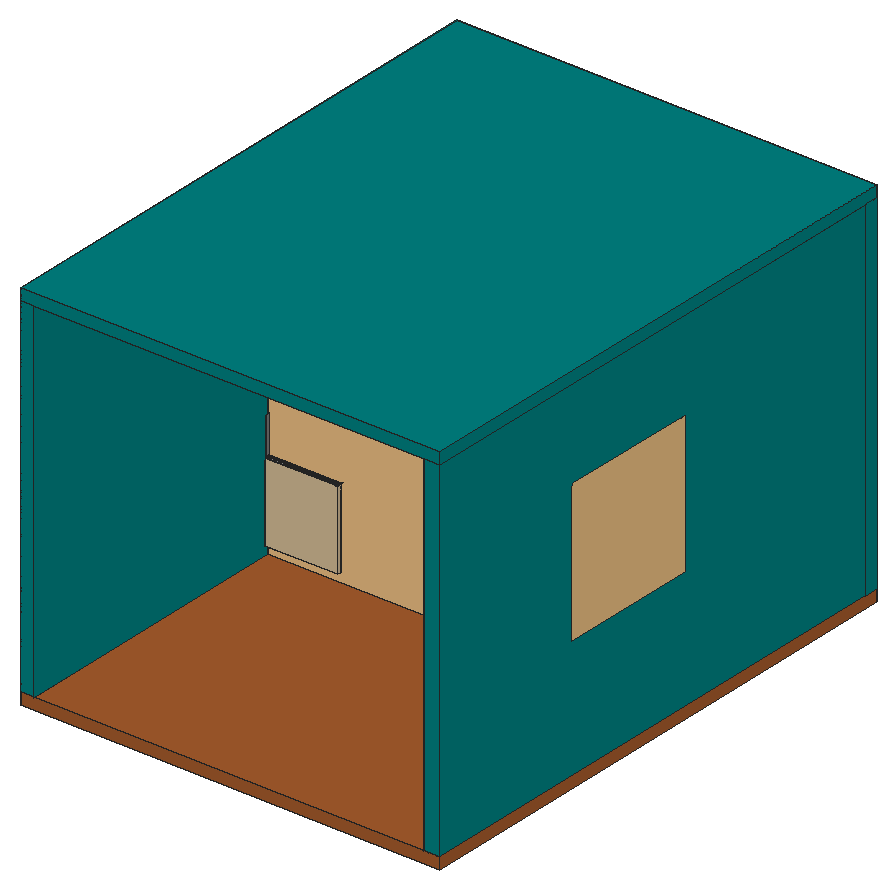
# SketchUp Ruby script. Lengths in inches.
U = 1.inch
M = Sketchup.active_model
def pt(a) = Geom::Point3d.new(a.map { |v| v * U })
def face(e, loops, mat)
  f = e.add_face(loops[0].map { |a| pt(a) })
  loops[1..].each { |l| e.add_face(l.map { |a| pt(a) }).erase! }
  f.material = f.back_material = mat if mat
  f
end
# faces: each face lists its corners as indices into pts; further lists are holes
def faces(e, pts, list, mat = nil) = list.each { |f| face(e, (f[0].is_a?(Array) ? f : [f]).map { |l| l.map { |i| pts[i] } }, mat) }
# xy, xz, yz: faces in a plane at the given z, y or x. An outline is a flat list of corners, or four numbers for a rectangle; further outlines are holes
def ring(l) = l.size == 4 ? [[l[0], l[1]], [l[2], l[1]], [l[2], l[3]], [l[0], l[3]]] : l.each_slice(2).to_a
def flat(e, list, mat, &to3) = list.each { |f| face(e, (f[0].is_a?(Array) ? f : [f]).map { |l| ring(l).map { |u, v| to3.(u, v) } }, mat) }
def xy(e, z, list, mat = nil) = flat(e, list, mat) { |x, y| [x, y, z] }
def xz(e, y, list, mat = nil) = flat(e, list, mat) { |x, z| [x, y, z] }
def yz(e, x, list, mat = nil) = flat(e, list, mat) { |y, z| [x, y, z] }
def lines(e, pts, list) = list.each { |a, b| e.add_line(pt(pts[a]), pt(pts[b])) }
# prism: a flat outline (further loops are holes) pulled along v
def prism(e, loops, v, mat = nil)
  f = face(e, loops, mat); d = Geom::Vector3d.new(v.map { |x| x * U })
  f.pushpull(f.normal.samedirection?(d) ? d.length : -d.length)
end
def box(e, o, s, mat = nil) = prism(e, [[o, [o[0] + s[0], o[1], o[2]], [o[0] + s[0], o[1] + s[1], o[2]], [o[0], o[1] + s[1], o[2]]]], [0, 0, s[2]], mat)
def at(x, y, z, deg = 0) = Geom::Transformation.translation(pt([x, y, z])) * Geom::Transformation.rotation(ORIGIN, Z_AXIS, deg.degrees)
def axes(o, x, y, z) = Geom::Transformation.new([*x, 0, *y, 0, *z, 0, *pt(o).to_a, 1])
def part(name) = M.definitions.add(name)
# library, detail: a bought-in or finely detailed component or shape, given as its bounding box
def library(name, o, s) = part(name).tap { |d| box(d.entities, o, s) }
def detail(e, o, s) = box(e.add_group.entities, o, s)
def put(e, d, t, mat = nil) = e.add_instance(d, t).tap { |i| i.material = mat if mat }
def group(e, t, mat = nil) = e.add_group.tap { |g| g.transformation = t; g.material = mat if mat }.entities
root = M.entities
M.materials.add("CLC2-PC-Blanc INTER").color = [249, 249, 249]
M.materials.add("Material \#1").color = [0, 0, 0]
M.materials.add("Standardmaterial30").color = [86, 86, 86]
M.materials.add("[0031_PapayaWhip]").color = [199, 195, 183]
M.materials.add("[0031_PapayaWhip]1").color = [211, 117, 3]
M.materials.add("[0079_Teal]").color = [0, 128, 128]
M.materials.add("[0088_Aquamarine]").color = [127, 255, 212]
M.materials.add("[0091_MintCream]").color = [201, 113, 3]
M.materials.add("[0099_LightSteelBlue]").color = [176, 196, 222]
M.materials.add("[Blacktop Old 01]").color = [132, 136, 139]
M.materials.add("[Blinds Wood White]").color = [138, 137, 139]
M.materials.add("[Encaustic Tile Circular 01]").color = [123, 123, 122]
M.materials.add("[Formica Beige]").color = [211, 187, 149]
M.materials.add("[Ornate Tile 01]").color = [202, 202, 202]
M.materials.add("[Resin Turquoise]").color = [117, 218, 223]
M.materials.add("[Stone Marble]").color = [143, 138, 136]
M.materials.add("[Stone Vein Gray]").color = [166, 165, 165]
M.materials.add("[Terrazzo Light Blue]").color = [196, 214, 227]
M.materials.add("[Tile Hexagon White]").color = [213, 206, 204]
M.materials.add("[Translucent Glass Gray]").color = [128, 128, 128]
M.materials["[Translucent Glass Gray]"].alpha = 0.5
M.materials.add("[Wood Board Cork]").color = [215, 201, 115]
M.materials.add("[Wood Cherry Original]").color = [152, 86, 42]
M.materials.add("[Wood Square Tile 01]").color = [164, 91, 44]
M.materials.add("utensils_wood_2").color = [89, 58, 24]
c1 = library("Group\#12",[-32.31,-359.75,0.0625],[113.14,110.83,100])
c2 = library("Group\#19",[-370.5625,-274.21,5.8125],[90.77,166.34,120.375])
c3 = library("Group\#17",[-278.11,-348.23,5.8],[187.87,187.87,121.65])
c4 = library("Group\#13",[-77.16,-243.45,0.06],[77.78,77.39,334.5])
c5 = library("Group\#11",[5.16,-238.13,0.06],[77.38,77.77,330.87])
c6 = library("Group\#21",[162.6875,-473.8,0.53],[157.34,166.37,329.78])
c7 = library("Group\#14",[-424.81,-54.29,0.29],[386.66,43.55,222.03])
c8 = library("Group\#20",[70.49,-356.56,0.0625],[143.03,166.7,314.72])
c9 = library("Group\#22",[-91.3125,-441.93,-0.01],[120,70.11,138.07])
c10 = library("Group\#16",[-375.96,-353.73,0.05],[297.45,297.44,31.27])
c11 = library("Group\#18",[-284.5,-166.25,5.875],[106.63,106.63,250.48])
c12 = part("Kitchen countertop accessories")
p = [[424.81,473.8,0.01],[425.81,473.8,0.01],[425.81,474.8,0.01]]
lines(c12.entities,p,[[0,1],[2,0]])
put(c12.entities,c1,at(424.81,473.8,0.01))
put(c12.entities,c2,at(424.81,473.8,0.01))
put(c12.entities,c3,at(424.81,473.8,0.01))
put(c12.entities,c4,at(424.81,473.8,0.01))
put(c12.entities,c5,at(424.81,473.8,0.01))
put(c12.entities,c6,at(424.81,473.8,0.01))
put(c12.entities,c7,at(424.81,473.8,0.01),"utensils_wood_2")
put(c12.entities,c8,at(424.81,473.8,0.01))
put(c12.entities,c9,at(424.81,473.8,0.01))
put(c12.entities,c10,at(424.81,473.8,0.01))
put(c12.entities,c11,at(424.81,473.8,0.01))
c13 = library("pellawindow\#4",[0,-3.05,0],[47.5,4.65,53.5])
c14 = library("007",[-28.95,-65.99,21.26],[5.48,1.13,0.69])
c15 = library("5-HOTTE ASPIRANTE CLC2",[-15.16,-17.72,-0.29],[30.34,17.72,30.09])
c16 = library("Hob1",[-15.52,-17.72,0],[31.04,35.44,3.4])
c17 = library("6-FOUR H60 CLC2",[0,-1.15,0],[23.5,21.54,23.5])
c18 = library("2-TABLE DE CUISSON CLC2",[-11.42,-10.04,0],[22.84,20.08,1.26])
c19 = part("CLC2-Ele02")
prism(c19.entities,[[[0.84,-0.32,0.16],[0.84,-0.33,0.02],[0.84,-0.34,-0.125],[0.84,-0.36,-0.27],[0.84,-0.39,-0.41],[0.84,-0.43,-0.55],[0.84,-0.47,-0.68],[0.84,-0.51,-0.82],[0.84,-0.2,-0.84],[0.84,-0.07,0.84],[0.84,-0.375,0.87],[0.84,-0.35,0.73],[0.84,-0.33,0.59],[0.84,-0.32,0.44],[0.84,-0.32,0.3]]],[-0.83,0,0],"CLC2-PC-Blanc INTER")
prism(c19.entities,[[[-0.01,-0.32,0.16],[-0.01,-0.33,0.02],[-0.01,-0.34,-0.125],[-0.01,-0.36,-0.27],[-0.01,-0.39,-0.41],[-0.01,-0.43,-0.55],[-0.01,-0.47,-0.68],[-0.01,-0.51,-0.82],[-0.01,-0.2,-0.84],[-0.01,-0.07,0.84],[-0.01,-0.375,0.87],[-0.01,-0.35,0.73],[-0.01,-0.33,0.59],[-0.01,-0.32,0.44],[-0.01,-0.32,0.3]]],[-0.83,0,0],"CLC2-PC-Blanc INTER")
xy(c19.entities,-1.57,[[-1.44,-0.19,1.44,0]],"CLC2-PC-Blanc INTER")
xy(c19.entities,-1.5,[[-1.375,-0.12,1.375,0]],"CLC2-PC-Blanc INTER")
xy(c19.entities,-0.87,[[-0.85,-0.29,0.85,-0.12]],"CLC2-PC-Blanc INTER")
xy(c19.entities,0.87,[[-0.85,-0.29,0.85,-0.12]],"CLC2-PC-Blanc INTER")
xy(c19.entities,1.5,[[-1.375,-0.12,1.375,0]],"CLC2-PC-Blanc INTER")
xy(c19.entities,1.57,[[-1.44,-0.19,1.44,0]],"CLC2-PC-Blanc INTER")
xz(c19.entities,-0.12,[[[-1.375,-1.5,-1.41,-1.3,-1.4375,-1.04,-1.46,-0.78,-1.48,-0.52,-1.5,0,-1.48,0.52,-1.46,0.78,-1.4375,1.04,-1.41,1.3,-1.375,1.5,1.375,1.5,1.41,1.3,1.4375,1.04,1.46,0.78,1.48,0.52,1.5,0,1.48,-0.52,1.46,-0.78,1.4375,-1.04,1.41,-1.3,1.375,-1.5],[-0.85,-0.87,0.85,0.87]]],"CLC2-PC-Blanc INTER")
xz(c19.entities,0,[[-1.44,-1.57,-1.48,-1.3125,-1.51,-1.05,-1.54,-0.79,-1.56,-0.53,-1.57,-0.26,-1.57,0.26,-1.56,0.53,-1.54,0.79,-1.51,1.05,-1.48,1.3125,-1.44,1.57,0,1.57,0,1.5,-1.375,1.5,-1.41,1.3,-1.4375,1.04,-1.46,0.78,-1.48,0.52,-1.5,0,-1.48,-0.52,-1.46,-0.78,-1.4375,-1.04,-1.41,-1.3,-1.375,-1.5,0,-1.5,0,-1.57],[0,-1.57,0,-1.5,1.375,-1.5,1.41,-1.3,1.4375,-1.04,1.46,-0.78,1.48,-0.52,1.5,0,1.48,0.52,1.46,0.78,1.4375,1.04,1.41,1.3,1.375,1.5,0,1.5,0,1.57,1.44,1.57,1.48,1.3125,1.51,1.05,1.54,0.79,1.56,0.53,1.57,0.26,1.57,-0.26,1.56,-0.53,1.54,-0.79,1.51,-1.05,1.48,-1.3125,1.44,-1.57]],"CLC2-PC-Blanc INTER")
yz(c19.entities,-1.57,[[-0.0625,-0.26,-0.06,0,0,0,0,-0.26],[-0.06,0,-0.0625,0.26,0,0.26,0,0]],"CLC2-PC-Blanc INTER")
yz(c19.entities,-0.85,[[-0.29,-0.87,-0.12,-0.87,-0.12,0.87,-0.29,0.87,-0.29,0.79,-0.3125,0.53,-0.32,0.26,-0.33,0,-0.32,-0.26,-0.3125,-0.53,-0.29,-0.79]],"CLC2-PC-Blanc INTER")
yz(c19.entities,0.85,[[-0.29,-0.87,-0.29,-0.79,-0.3125,-0.53,-0.32,-0.26,-0.33,0,-0.32,0.26,-0.3125,0.53,-0.29,0.79,-0.29,0.87,-0.12,0.87,-0.12,-0.87]],"CLC2-PC-Blanc INTER")
yz(c19.entities,1.57,[[-0.0625,-0.26,0,-0.26,0,0,-0.06,0],[-0.06,0,0,0,0,0.26,-0.0625,0.26]],"CLC2-PC-Blanc INTER")
p = [[-1.32,-0.3125,0.53],[-1.34,-0.29,0.79],[-1.37,-0.27,1.05],[-1.4,-0.23,1.3125],[-1.44,-0.19,1.57],[-1.48,-0.15,1.3125],
  [-1.51,-0.12,1.05],[-1.54,-0.09,0.79],[-1.56,-0.07,0.53],[-1.57,-0.0625,0.26],[-1.57,-0.06,0],[-1.57,-0.0625,-0.26],
  [-1.56,-0.07,-0.53],[-1.54,-0.09,-0.79],[-1.51,-0.12,-1.05],[-1.48,-0.15,-1.3125],[-1.44,-0.19,-1.57],[-1.4,-0.23,-1.3125],
  [-1.37,-0.27,-1.05],[-1.34,-0.29,-0.79],[-1.32,-0.3125,-0.53],[-1.31,-0.32,-0.26],[-1.3,-0.33,0],[-1.31,-0.32,0.26],
  [1.34,-0.29,0.79],[1.32,-0.3125,0.53],[1.31,-0.32,0.26],[1.3,-0.33,0],[1.31,-0.32,-0.26],[1.32,-0.3125,-0.53],
  [1.34,-0.29,-0.79],[1.37,-0.27,-1.05],[1.4,-0.23,-1.3125],[1.44,-0.19,-1.57],[1.48,-0.15,-1.3125],[1.51,-0.12,-1.05],
  [1.54,-0.09,-0.79],[1.56,-0.07,-0.53],[1.57,-0.0625,-0.26],[1.57,-0.06,0],[1.57,-0.0625,0.26],[1.56,-0.07,0.53],
  [1.54,-0.09,0.79],[1.51,-0.12,1.05],[1.48,-0.15,1.3125],[1.44,-0.19,1.57],[1.4,-0.23,1.3125],[1.37,-0.27,1.05],
  [-1.44,0,-1.57],[-1.48,0,-1.3125],[1.44,0,-1.57],[1.48,0,-1.3125],[-1.375,0,-1.5],[-1.41,0,-1.3],
  [-1.41,-0.12,-1.3],[-1.375,-0.12,-1.5],[1.41,0,-1.3],[1.375,0,-1.5],[1.375,-0.12,-1.5],[1.41,-0.12,-1.3],
  [-1.51,0,-1.05],[1.51,0,-1.05],[-1.4375,0,-1.04],[-1.4375,-0.12,-1.04],[1.4375,0,-1.04],[1.4375,-0.12,-1.04],
  [0.85,-0.29,-0.87],[-0.85,-0.29,-0.87],[-0.85,-0.29,-0.79],[-1.33,-0.29,-0.79],[1.33,-0.29,-0.79],[0.85,-0.29,-0.79],
  [-1.54,0,-0.79],[1.54,0,-0.79],[-1.46,0,-0.78],[-1.46,-0.12,-0.78],[1.46,0,-0.78],[1.46,-0.12,-0.78],
  [-0.85,-0.3125,-0.53],[0.85,-0.3125,-0.53],[-1.56,0,-0.53],[-1.48,0,-0.52],[-1.48,-0.12,-0.52],[1.48,0,-0.52],
  [1.48,-0.12,-0.52],[1.56,0,-0.53],[-0.85,-0.32,-0.26],[0.85,-0.32,-0.26],[-1.57,0,-0.26],[-1.49,0,-0.26],
  [-1.49,-0.12,-0.26],[1.49,0,-0.26],[1.49,-0.12,-0.26],[1.57,0,-0.26],[-0.85,-0.33,0],[0.85,-0.33,0],
  [-1.5,0,0],[-1.5,-0.12,0],[1.5,0,0],[1.5,-0.12,0],[-0.85,-0.32,0.26],[0.85,-0.32,0.26],
  [-1.49,0,0.26],[-1.49,-0.12,0.26],[1.49,0,0.26],[1.49,-0.12,0.26],[-0.85,-0.3125,0.53],[0.85,-0.3125,0.53],
  [-1.57,0,0.26],[-1.56,0,0.53],[-1.48,0,0.52],[-1.48,-0.12,0.52],[1.48,0,0.52],[1.48,-0.12,0.52],
  [1.57,0,0.26],[1.56,0,0.53],[-0.85,-0.29,0.79],[-1.33,-0.29,0.79],[1.33,-0.29,0.79],[0.85,-0.29,0.79],
  [-1.54,0,0.79],[-1.46,0,0.78],[-1.46,-0.12,0.78],[1.46,0,0.78],[1.46,-0.12,0.78],[1.54,0,0.79],
  [-0.85,-0.29,0.87],[0.85,-0.29,0.87],[-1.4375,0,1.04],[-1.4375,-0.12,1.04],[-1.51,0,1.05],[1.4375,0,1.04],
  [1.4375,-0.12,1.04],[1.51,0,1.05],[-1.41,0,1.3],[-1.41,-0.12,1.3],[1.41,0,1.3],[1.41,-0.12,1.3],
  [-1.48,0,1.3125],[1.48,0,1.3125],[-1.44,0,1.57],[1.44,0,1.57],[-1.375,0,1.5],[-1.375,-0.12,1.5],
  [1.375,0,1.5],[1.375,-0.12,1.5]]
faces(c19.entities,p,[[0,1,2,3,4,5,6,7,8,9,10,11,12,13,14,15,16,17,18,19,20,21,22,23],[24,25,26,27,28,29,30,31,32,33,34,35,36,37,38,39,40,41,42,43,44,45,46,47],[48,16,15,49],[32,17,16,33],[33,50,51,34],[52,53,54,55],[56,57,58,59],[31,18,17,32],
  [49,15,14,60],[34,51,61,35],[53,62,63,54],[64,56,59,65],[66,67,68,69,19,18,31,30,70,71],[60,14,13,72],[35,61,73,36],[62,74,75,63],
  [76,64,65,77],[69,68,78,20,19],[71,70,30,29,79],[72,13,12,80],[74,81,82,75],[83,76,77,84],[36,73,85,37],[20,78,86,21],
  [79,29,28,87],[80,12,11,88],[81,89,90,82],[91,83,84,92],[37,85,93,38],[21,86,94,22],[87,28,27,95],[89,96,97,90],
  [98,91,92,99],[22,94,100,23],[95,27,26,101],[96,102,103,97],[104,98,99,105],[23,100,106,0],[101,26,25,107],[108,9,8,109],
  [102,110,111,103],[112,104,105,113],[40,114,115,41],[0,106,116,117,1],[107,25,24,118,119],[109,8,7,120],[110,121,122,111],[123,112,113,124],
  [41,115,125,42],[116,126,127,119,118,24,47,2,1,117],[121,128,129,122],[120,7,6,130],[131,123,124,132],[42,125,133,43],[128,134,135,129],[136,131,132,137],
  [46,3,2,47],[130,6,5,138],[43,133,139,44],[138,5,4,140],[4,3,46,45],[44,139,141,45],[134,142,143,135],[144,136,137,145]],"CLC2-PC-Blanc INTER")
c20 = part("2-PRISEELC CLC2")
put(c20.entities,c19,axes([0,0,0],[1,0,0],[0,0,-1],[0,1,0]))
c21 = library("15-PRODUITS CUISINE CLC2",[-1.94,-2.15,0],[3.93,3.94,5.51])
c22 = library("12-PRODUITS CUISINE CLC2",[-1.08,-1.08,0],[2.16,2.16,5.375])
c23 = library("15-PRODUITS CUISINE CLC2\#1",[-1.94,-2.15,0],[3.93,3.94,5.51])
c24 = library("Kitchen sink with faucet",[-0.15,-0.12,-6.4],[37.85,20.23,20.6])
c25 = library("AS-120-mm",[0,0,0],[48,4.72,48])
c26 = library("9-POIGNEE CLC2",[-3.01,-0.26,0],[6.02,0.52,1.49])
c27 = library("2-POIGNEE CLC2",[-2.66,-0.49,0],[5.32,0.98,1.3])
c28 = library("Group\#4",[0,32.625,0],[131,82,57])
c29 = part("Union")
xy(c29.entities,0,[[0,51.67,0.1,82.93]],"[Tile Hexagon White]")
xy(c29.entities,0.04,[[0.1875,0,0,51.67,0.1,51.67,0.29,0]],"[Tile Hexagon White]")
xy(c29.entities,12.44,[[0.1875,0,0.29,0,0.1,51.67,0,51.67]],"[Tile Hexagon White]")
xy(c29.entities,29.375,[[0,51.67,0.1,82.93]],"[Tile Hexagon White]")
xz(c29.entities,0,[[0.1875,0.04,0.29,12.44]],"[Tile Hexagon White]")
xz(c29.entities,51.67,[[0,0,0.1,0.04],[0,12.44,0.1,29.375]],"[Tile Hexagon White]")
xz(c29.entities,82.93,[[0,0,0.1,29.375]],"[Tile Hexagon White]")
yz(c29.entities,0,[[51.67,0,82.93,29.375]],"[Tile Hexagon White]")
yz(c29.entities,0.1,[[51.67,0,82.93,29.375]],"[Encaustic Tile Circular 01]")
p = [[0,51.67,0.04],[0.1875,0,0.04],[0.1875,0,12.44],[0,51.67,12.44],[0.29,0,0.04],[0.1,51.67,0.04],
  [0.1,51.67,12.44],[0.29,0,12.44]]
faces(c29.entities,p,[[0,1,2,3]],"[Tile Hexagon White]")
faces(c29.entities,p,[[4,5,6,7]],"[Encaustic Tile Circular 01]")
c30 = part("Group\#39")
box(c30.entities,[0,-0.16,0],[14.04,0.16,8.44])
c31 = library("Group\#36",[0,0,0],[13.37,2.97,7.55])
c32 = part("Union\#1")
xy(c32.entities,0,[[0,48.27,0.1,124.86]])
xy(c32.entities,0,[[0,0,0.1,48.27]],"[Encaustic Tile Circular 01]")
xy(c32.entities,10.36,[[0,0,0.1,47.52]],"[Encaustic Tile Circular 01]")
xy(c32.entities,29.13,[[0,47.52,0.1,124.86]])
xz(c32.entities,0,[[0,0,0.1,10.36]],"[Encaustic Tile Circular 01]")
xz(c32.entities,47.52,[[0,10.36,0.1,29.13]])
xz(c32.entities,124.86,[[0,0,0.1,29.13]])
yz(c32.entities,0,[[0,0,0,10.36,47.52,10.36,47.52,29.13,124.86,29.13,124.86,0]],"[Encaustic Tile Circular 01]")
yz(c32.entities,0.1,[[48.27,0,124.86,0,124.86,29.13,47.52,29.13,47.52,10.36,48.27,10.36]])
yz(c32.entities,0.1,[[0,0,48.27,10.36]],"[Encaustic Tile Circular 01]")
c33 = library("Group\#182",[0,0,0],[42.16,31.84,40.44])
c34 = library("Group\#184",[0,0,-7.25],[98.84,110.93,7.25])
xz(root,161.23,[[99.375,31.2,126.76,31.21]],"[Stone Vein Gray]")
xz(root,176.99,[[99.375,31.2,126.76,31.21]],"[Stone Vein Gray]")
yz(root,99.375,[[161.23,31.2,176.99,31.21]],"[Stone Vein Gray]")
p = [[29.43,157.1875,3],[29.43,157.1875,30],[126.76,161.23,31.2],[126.76,176.99,31.2],[0,18.6875,120],[0,186.6875,120],
  [143.41,186.6875,120],[143.41,18.6875,120]]
lines(root,p,[[0,1],[2,3],[4,5],[5,6],[6,7],[7,4]])
put(root,c12,axes([19.84,158.83,30.625],[0,0.0275,0],[-0.0275,0,0],[0,0,0.0275]))
put(root,c13,at(1.5,102.92,42.625,90))
put(root,c14,axes([77.75,192.75,48.53],[0,0,0.87],[0,0.5481,0],[-0.87,0,0]))
put(root,c14,axes([71.76,192.75,48.53],[0,0,0.87],[0,0.5481,0],[-0.87,0,0]))
put(root,c14,axes([53.76,192.74,48.77],[0,0,0.87],[0,0.5481,0],[-0.87,0,0]))
put(root,c14,axes([95.6,192.75,52.97],[0,0,0.87],[0,0.5481,0],[-0.87,0,0]))
put(root,c14,axes([113.81,192.75,48.53],[0,0,0.87],[0,0.5481,0],[-0.87,0,0]))
put(root,c14,axes([141.37,192.75,48.53],[0,0,0.87],[0,0.5481,0],[-0.87,0,0]))
put(root,c14,axes([143.24,192.75,48.53],[0,0,0.87],[0,0.5481,0],[-0.87,0,0]))
put(root,c14,axes([-6.01,115.6,38.68],[0,-0.87,0],[-0.5481,0,0],[0,0,-0.87]))
put(root,c14,axes([-6.05,129.48,46.95],[0,0,0.87],[-0.5481,0,0],[0,-0.87,0]))
put(root,c14,axes([-6.05,132.24,46.95],[0,0,0.87],[-0.5481,0,0],[0,-0.87,0]))
put(root,c14,axes([-6.05,115.6,44.93],[0,-0.87,0],[-0.5481,0,0],[0,0,-0.87]))
put(root,c14,axes([-5.95,115.6,33.24],[0,-0.87,0],[-0.5481,0,0],[0,0,-0.87]))
put(root,c15,axes([6.52,134.6875,76.78],[0.00015,0.99911,0.01208],[-0.99993,0,0.01209],[0.01595,-0.01595,1.31981]))
put(root,c16,axes([16.75,138.99,30.625],[0.68089,0,0],[0,0.79341,0],[0,0,1.1662]),"Material \#1")
put(root,c17,axes([51.02,159.49,30.625],[1,0,0],[0,1,0],[0,0,1.05]))
put(root,c18,at(16.86,138.26,30.625))
put(root,c20,axes([18.77,181.49,47.7],[1,0,0],[0,0,1],[0,-1,0]))
put(root,c21,axes([75.13,173.46,72.5],[1.17,0,0],[0,1.17,0],[0,0,1.07359]))
put(root,c22,axes([85.96,170.82,72.5],[1.17,0,0],[0,1.17,0],[0,0,1.07359]))
put(root,c23,axes([79.76,173.46,72.5],[1.17,0,0],[0,1.17,0],[0,0,1.07359]))
put(root,c22,axes([83.6,173.46,72.5],[1.17,0,0],[0,1.17,0],[0,0,1.07359]))
put(root,c24,axes([96.12,161.06,31.38],[1,0,0],[0,1,-0.00308],[0,0.00308,1]))
put(root,c25,at(143.41,56.625,41.24,90))
put(root,c26,axes([18.44,167.1875,73.7],[1,0,0],[0,0,0.99928],[0,-1.00073,0]))
put(root,c26,axes([18.44,167.1875,61.05],[1,0,0],[0,0,0.99928],[0,-1.00073,0]))
put(root,c26,axes([122.88,167.1875,73.7],[1,0,0],[0,0,0.99928],[0,-1.00073,0]))
put(root,c26,axes([122.88,167.1875,61.05],[1,0,0],[0,0,0.99928],[0,-1.00073,0]))
put(root,c27,axes([37.15,167.1875,73.34],[0,0,1],[-1,0,0],[0,-1,0]))
put(root,c27,axes([91.29,167.1875,73.34],[0,0,1],[-1,0,0],[0,-1,0]))
put(root,c28,at(4.5,67.5625,0),"[Terrazzo Light Blue]")
g1 = group(root,at(4.5,182.1875,60),"[Wood Board Cork]")
xy(g1,0,[[1,-14,49.09,0],[85.16,-14,133,0]],"[Wood Board Cork]")
xy(g1,11.5,[[49.09,-14,85.16,0]],"[Wood Board Cork]")
xy(g1,12.5,[[50.09,-14,84.16,-0.75]],"[0031_PapayaWhip]")
xy(g1,22.94,[[50.09,-14,84.16,-0.75]],"[0031_PapayaWhip]")
xy(g1,23.94,[[1,-14,49.09,0],[49.09,-14,85.16,0],[85.16,-14,133,0]],"[Wood Board Cork]")
xz(g1,-14,[[1,0,49.09,23.94],[85.16,0,133,23.94],[[49.09,11.5,85.16,23.94],[50.09,12.5,84.16,22.94]]],"[0031_PapayaWhip]")
xz(g1,-0.75,[[50.09,12.5,84.16,22.94]],"[0031_PapayaWhip]")
xz(g1,0,[[1,0,1,23.94,133,23.94,133,0,85.16,0,85.16,11.5,49.09,11.5,49.09,0]],"[0031_PapayaWhip]")
yz(g1,1,[[-14,0,0,23.94]],"[0031_PapayaWhip]")
yz(g1,49.09,[[-14,0,0,11.5]],"[Wood Board Cork]")
yz(g1,84.16,[[-14,12.5,-0.75,22.94]],"[0031_PapayaWhip]")
yz(g1,85.16,[[-14,0,0,11.5]],"[Wood Board Cork]")
yz(g1,133,[[-14,0,0,23.94]],"[0031_PapayaWhip]")
g2 = group(g1,at(50.09,-14,12.5))
yz(g2,0,[[0,0,13.25,10.44]])
g3 = group(root,at(4.5,168.1875,60),"[Blinds Wood White]")
box(g3,[31.16,-1,0],[17.93,1,23.94],"[0031_PapayaWhip]")
xy(g3,0,[[85.16,-1,103,0]],"[0031_PapayaWhip]")
xy(g3,23.94,[[85.16,-1,103,0]],"[0031_PapayaWhip]")
xz(g3,-1,[[85.16,0,103,23.94]],"[0031_PapayaWhip]")
xz(g3,0,[[85.16,0,103,23.94]],"[0031_PapayaWhip]")
yz(g3,85.16,[[-1,0,0,23.94]],"[0031_PapayaWhip]")
yz(g3,103,[[-1,0,0,23.94]],"[0031_PapayaWhip]")
p = [[84,-0.34,22.94],[84,-0.54,22.94]]
lines(g3,p,[[0,1]])
g4 = group(g3,at(0,-1,0),"[Wood Board Cork]")
xy(g4,0,[[0,0,1,15],[1,0,31,1]],"[Wood Board Cork]")
xy(g4,11.89,[[1,0,31,1]],"[Wood Board Cork]")
xy(g4,12.05,[[1,0,31,1]],"[0091_MintCream]")
xy(g4,23.94,[[0,0,1,15],[1,0,31,1]],"[Wood Board Cork]")
xz(g4,0,[[0,0,1,23.94],[1,0,31,11.89],[1,12.05,31,23.94]],"[Wood Board Cork]")
xz(g4,1,[[1,0,31,11.89],[1,11.89,31,12.05],[1,12.05,31,23.94]],"[0091_MintCream]")
xz(g4,15,[[0,0,1,23.94]],"[0091_MintCream]")
yz(g4,0,[[0,0,15,23.94]],"[0091_MintCream]")
yz(g4,1,[[0,0,1,11.89],[1,0,15,23.94],[0,11.89,1,12.05],[0,12.05,1,23.94]],"[0091_MintCream]")
yz(g4,31,[[0,0,1,11.89],[0,12.05,1,23.94]],"[Wood Board Cork]")
g5 = group(g3,at(103.16,-1,12.05),"[Wood Board Cork]")
xy(g5,0,[[0,0,29.84,1]],"[0031_PapayaWhip]1")
xy(g5,11.89,[[0,0,29.84,1]],"[Wood Board Cork]")
xz(g5,0,[[0,0,29.84,11.89]],"[Wood Board Cork]")
xz(g5,1,[[0,0,29.84,11.89]],"[0031_PapayaWhip]1")
yz(g5,0,[[0,0,1,11.89]],"[Wood Board Cork]")
yz(g5,29.84,[[0,0,1,11.89]],"[Wood Board Cork]")
g6 = group(g3,at(103.16,-1,0),"[Wood Board Cork]")
xy(g6,0,[[0,0,29.84,1]],"[Wood Board Cork]")
xy(g6,11.89,[[0,0,29.84,1]],"[Wood Board Cork]")
xz(g6,0,[[0,0,29.84,11.89]],"[Wood Board Cork]")
xz(g6,1,[[0,0,29.84,11.89]],"[Wood Cherry Original]")
yz(g6,0,[[0,0,1,11.89]],"[Wood Cherry Original]")
yz(g6,29.84,[[0,0,1,11.89]],"[Wood Board Cork]")
g7 = group(g3,at(133.16,-1,0),"[Wood Board Cork]")
xy(g7,0,[[0,0,2.25,15]],"[Wood Board Cork]")
xy(g7,23.94,[[0,0,2.25,15]],"[Wood Board Cork]")
xz(g7,0,[[0,0,2.25,23.94]],"[Wood Board Cork]")
xz(g7,15,[[0,0,2.25,23.94]],"[Wood Cherry Original]")
yz(g7,0,[[0,0,1,23.94],[1,0,15,23.94]],"[Wood Cherry Original]")
yz(g7,2.25,[[0,0,15,23.94]],"[Wood Board Cork]")
g8 = group(root,at(54.59,168.1875,72.5))
box(g8,[-1,0,0],[1,13.25,10.44])
g9 = group(root,at(28.5,67.5625,3),"[Formica Beige]")
box(g9,[0,56.625,0],[1,29.84,13.54])
box(g9,[0,56.625,20.35],[1,29.84,6.65])
box(g9,[0,56.625,13.62],[1,29.84,6.65])
xy(g9,0,[[0,32.625,1,44.42],[0,44.58,1,56.47]])
xy(g9,0,[[-24,31.5,1,32.47]],"[Terrazzo Light Blue]")
xy(g9,26.1,[[0.125,32.72,1,44.32],[0.125,44.68,1,56.37]],"Standardmaterial30")
xy(g9,26.78,[[0.5625,32.72,1,44.32],[0.57,44.68,1,56.37]],"Standardmaterial30")
xy(g9,26.9,[[0.125,32.72,0.5625,44.32],[0.125,44.68,0.57,56.37]])
xy(g9,27,[[0,32.625,1,44.42],[0,44.58,1,56.47]])
xy(g9,27,[[-24,31.5,1,32.47]],"[Terrazzo Light Blue]")
xz(g9,31.5,[[-24,0,1,27]],"[Formica Beige]")
xz(g9,32.47,[[-24,0,1,27]],"[Terrazzo Light Blue]")
xz(g9,32.625,[[0,0,1,27]])
xz(g9,32.72,[[0.125,26.1,0.125,26.9,0.5625,26.9,0.5625,26.78,1,26.78,1,26.1]],"Standardmaterial30")
xz(g9,44.32,[[0.125,26.1,1,26.1,1,26.78,0.5625,26.78,0.5625,26.9,0.125,26.9]],"Standardmaterial30")
xz(g9,44.42,[[0,0,1,27]])
xz(g9,44.58,[[0,0,1,27]])
xz(g9,44.68,[[0.125,26.1,0.125,26.9,0.57,26.9,0.57,26.78,1,26.78,1,26.1]],"Standardmaterial30")
xz(g9,56.37,[[0.125,26.1,1,26.1,1,26.78,0.57,26.78,0.57,26.9,0.125,26.9]],"Standardmaterial30")
xz(g9,56.47,[[0,0,1,27]])
yz(g9,-24,[[31.5,0,32.47,27]],"[Terrazzo Light Blue]")
yz(g9,0,[[32.625,0,44.42,27],[44.42,0,44.58,27],[44.58,0,56.47,27]])
yz(g9,0.125,[[32.72,26.1,44.32,26.9],[44.68,26.1,56.37,26.9]],"Standardmaterial30")
yz(g9,0.5625,[[32.72,26.78,44.32,26.9]])
yz(g9,0.57,[[44.68,26.78,56.37,26.9]])
yz(g9,1,[[[32.625,26,44.42,27],[32.72,26.1,44.32,26.78]],[[44.58,26,56.47,27],[44.68,26.1,56.37,26.78]]])
yz(g9,1,[[31.5,0,32.47,27],[32.625,0,44.42,26],[44.58,0,56.47,26]],"[Formica Beige]")
g10 = group(g9,at(0,86.625,0))
prism(g10,[[[1,3,0],[1,0,0],[0,0,0],[0,4,0],[1,4,0]]],[0,0,27])
g11 = group(root,at(29.5,157.1875,3),"[Stone Marble]")
xy(g11,0,[[22.16,0,28,1],[28.16,0,46,1],[64.16,0,82,1],[82.16,0,94,1],[94.16,0,106,1],
  [106.16,0,108.22,25]])
xy(g11,0,[[4.16,0,22,1]],"[Terrazzo Light Blue]")
xy(g11,27,[[22.16,0,28,1],[28.16,0,46,1],[64.16,0,82,1],[82.16,0,94,1],[94.16,0,106,1]])
xy(g11,27,[[4.16,0,22,1],[106.16,0,108.22,25]],"[Terrazzo Light Blue]")
xz(g11,0,[[4.16,0,22,27],[22.16,0,28,27],[28.16,0,46,27],[64.16,0,82,27],[82.16,0,94,27],
  [94.16,0,106,27],[106.16,0,108.22,27]],"[Formica Beige]")
xz(g11,1,[[22.16,0,28,27],[28.16,0,46,27],[64.16,0,82,27],[82.16,0,94,27],[94.16,0,106,27]])
xz(g11,1,[[4.16,0,22,27]],"[Terrazzo Light Blue]")
xz(g11,25,[[106.16,0,108.22,27]])
yz(g11,4.16,[[0,0,1,27]],"[Terrazzo Light Blue]")
yz(g11,22,[[0,0,1,27]],"[Terrazzo Light Blue]")
yz(g11,22.16,[[0,0,1,27]])
yz(g11,28,[[0,0,1,27]])
yz(g11,28.16,[[0,0,1,27]])
yz(g11,46,[[0,0,1,27]])
yz(g11,64.16,[[0,0,1,27]])
yz(g11,82,[[0,0,1,27]])
yz(g11,82.16,[[0,0,1,27]])
yz(g11,94,[[0,0,1,27]])
yz(g11,94.16,[[0,0,1,27]])
yz(g11,106,[[0,0,1,27]])
yz(g11,106.16,[[0,0,1,27],[1,0,25,27]])
yz(g11,108.22,[[0,0,25,27]],"[Formica Beige]")
g12 = group(g11,at(0,0,0),"[Formica Beige]")
box(g12,[0,0,0],[4,1,27])
g13 = group(root,at(75.5,158.1875,3),"[Formica Beige]")
prism(g13,[[[18.16,0,53.0625],[18.16,0,27],[18.16,0,0],[0,0,0],[0,0,27],[0,0,53.0625]]],[0,-1,0])
g14 = group(root,at(4.5,100.1875,30))
xy(g14,-0.22,[[0,-0.76,0,-0.72,24.6,-0.72,24.64,-0.76],[24.64,-0.76,24.6,-0.72,24.6,57.4,24.64,57.36],[0,-0.72,0,82,71,82,71,57.4,24.6,57.4,24.6,-0.72],[24.64,57.36,24.6,57.4,71,57.4,71,57.36]],"[Stone Vein Gray]")
xy(g14,0.625,[[0,-0.83,24.71,-0.83,24.67,-0.79,0,-0.79],[24.71,-0.83,24.71,57.29,24.67,57.33,24.67,-0.79],[0,-0.79,24.67,-0.79,24.67,57.33,71,57.33,71,82,0,82],[24.71,57.29,71,57.29,71,57.33,24.67,57.33]],"[Stone Vein Gray]")
xz(g14,-1.125,[[0,0,25,0.39]],"[Stone Vein Gray]")
xz(g14,57,[[25,0,71,0.39]],"[Stone Vein Gray]")
xz(g14,82,[[0,-0.22,71,0.625]],"[Stone Vein Gray]")
yz(g14,0,[[-0.76,-0.22,-0.92,-0.18,-0.95,-0.16,-0.99,-0.14,-1.02,-0.12,-1.05,-0.09,-1.08,-0.0625,-1.1,-0.03,-1.125,0,-1.125,0.39,-1.11,0.42,-1.05,0.51,-1,0.56,-0.97,0.58,-0.93,0.6,-0.87,0.62,-0.83,0.625,82,0.625,82,-0.22]],"[Stone Vein Gray]")
yz(g14,25,[[-1.125,0,57,0.39]],"[Stone Vein Gray]")
yz(g14,71,[[57.36,-0.22,82,-0.22,82,0.625,57.29,0.625,57.26,0.62,57.22,0.61,57.19,0.6,57.1,0.54,57.07,0.51,57.01,0.42,57,0.39,57,0,57.02,-0.03,57.05,-0.0625,57.08,-0.09,57.11,-0.12,57.17,-0.16,57.21,-0.18,57.24,-0.19]],"[Stone Vein Gray]")
p = [[0,-0.95,-0.16],[0,-0.92,-0.18],[24.79,-0.92,-0.18],[24.83,-0.95,-0.16],[0,-0.99,-0.14],[24.86,-0.99,-0.14],
  [24.79,57.21,-0.18],[24.83,57.17,-0.16],[24.86,57.14,-0.14],[0,-0.88,-0.19],[0,-0.84,-0.2],[24.72,-0.84,-0.2],
  [24.76,-0.88,-0.19],[24.72,57.28,-0.2],[24.76,57.24,-0.19],[0,-0.8,-0.21],[0,-0.76,-0.22],[24.64,-0.76,-0.22],
  [24.68,-0.8,-0.21],[24.64,57.36,-0.22],[24.68,57.32,-0.21],[71,57.17,-0.16],[71,57.14,-0.14],[71,57.28,-0.2],
  [71,57.24,-0.19],[71,57.21,-0.18],[71,57.36,-0.22],[71,57.32,-0.21],[0,-1.08,-0.0625],[0,-1.05,-0.09],
  [24.92,-1.05,-0.09],[24.95,-1.08,-0.0625],[0,-1.1,-0.03],[24.98,-1.1,-0.03],[24.92,57.08,-0.09],[24.95,57.05,-0.0625],
  [24.98,57.02,-0.03],[0,-1.02,-0.12],[24.89,-1.02,-0.12],[24.89,57.11,-0.12],[71,57.08,-0.09],[71,57.05,-0.0625],
  [71,57.02,-0.03],[71,57.11,-0.12],[0,-1.125,0],[25,-1.125,0],[25,57,0],[71,57,0],
  [0,-1.11,0.42],[0,-1.125,0.39],[25,-1.125,0.39],[24.99,-1.11,0.42],[0,-1.09,0.45],[24.97,-1.09,0.45],
  [25,57,0.39],[24.99,57.01,0.42],[24.97,57.03,0.45],[71,57,0.39],[71,57.01,0.42],[71,57.03,0.45],
  [0,-1.07,0.48],[24.95,-1.07,0.48],[0,-1.05,0.51],[24.93,-1.05,0.51],[0,-1.02,0.54],[24.9,-1.02,0.54],
  [24.95,57.05,0.48],[24.93,57.07,0.51],[24.9,57.1,0.54],[0,-1,0.56],[24.87,-1,0.56],[24.87,57.13,0.56],
  [71,57.05,0.48],[71,57.07,0.51],[71,57.1,0.54],[71,57.13,0.56],[0,-0.97,0.58],[24.84,-0.97,0.58],
  [0,-0.93,0.6],[24.81,-0.93,0.6],[24.84,57.16,0.58],[24.81,57.19,0.6],[0,-0.9,0.61],[24.78,-0.9,0.61],
  [0,-0.87,0.62],[24.74,-0.87,0.62],[0,-0.83,0.625],[24.71,-0.83,0.625],[24.78,57.22,0.61],[24.74,57.26,0.62],
  [24.71,57.29,0.625],[71,57.16,0.58],[71,57.22,0.61],[71,57.26,0.62],[71,57.19,0.6],[71,57.29,0.625],
  [71,82,0],[89.16,82,0],[89.16,58,0]]
faces(g14,p,[[0,1,2,3],[4,0,3,5],[3,2,6,7],[5,3,7,8],[9,10,11,12],[1,9,12,2],[12,11,13,14],[2,12,14,6],
  [15,16,17,18],[10,15,18,11],[18,17,19,20],[11,18,20,13],[8,7,21,22],[14,13,23,24],[6,14,24,25],[7,6,25,21],
  [20,19,26,27],[13,20,27,23],[28,29,30,31],[32,28,31,33],[31,30,34,35],[33,31,35,36],[37,4,5,38],[29,37,38,30],
  [38,5,8,39],[30,38,39,34],[35,34,40,41],[36,35,41,42],[39,8,22,43],[34,39,43,40],[44,32,33,45],[45,33,36,46],
  [46,36,42,47],[48,49,50,51],[52,48,51,53],[51,50,54,55],[53,51,55,56],[55,54,57,58],[56,55,58,59],[60,52,53,61],
  [62,60,61,63],[64,62,63,65],[61,53,56,66],[63,61,66,67],[65,63,67,68],[69,64,65,70],[70,65,68,71],[66,56,59,72],
  [67,66,72,73],[68,67,73,74],[71,68,74,75],[76,69,70,77],[78,76,77,79],[77,70,71,80],[79,77,80,81],[82,78,79,83],
  [84,82,83,85],[86,84,85,87],[85,83,88,89],[87,85,89,90],[83,79,81,88],[80,71,75,91],[89,88,92,93],[81,80,91,94],
  [88,81,94,92],[90,89,93,95]],"[Stone Vein Gray]")
lines(g14,p,[[96,97],[98,97]])
put(root,c29,at(4.5,99.25,30.625))
g15 = group(root,at(0,-53.3125,0),"[0088_Aquamarine]")
xy(g15,0,[[0,53.3125,0,240,143.41,240,143.41,235.5,4.5,235.5,4.5,53.3125]],"[0079_Teal]")
xy(g15,42.625,[[0,156.24,4.5,204.24]],"[0079_Teal]")
xy(g15,93.8125,[[0,156.24,4.5,204.24]],"[0079_Teal]")
xy(g15,120,[[0,53.3125,4.5,53.3125,4.5,235.5,143.41,235.5,143.41,240,0,240]],"[0079_Teal]")
xz(g15,53.3125,[[0,0,4.5,120]],"[0079_Teal]")
xz(g15,156.24,[[0,42.625,4.5,93.8125]],"[0079_Teal]")
xz(g15,204.24,[[0,42.625,4.5,93.8125]],"[0079_Teal]")
xz(g15,235.5,[[4.5,0,143.41,120]],"[0079_Teal]")
xz(g15,240,[[0,0,143.41,120]],"[0079_Teal]")
yz(g15,0,[[[53.3125,0,240,120],[156.24,42.625,204.24,93.8125]]],"[0079_Teal]")
yz(g15,4.5,[[[53.3125,0,235.5,120],[156.24,42.625,204.24,93.8125]]],"[0079_Teal]")
yz(g15,143.41,[[235.5,0,240,120]],"[0079_Teal]")
g16 = group(root,at(0,-53.3125,-4))
box(g16,[0,53.3125,0],[143.41,186.6875,4],"[Wood Square Tile 01]")
g17 = group(root,at(70.84,168.1875,72.5))
box(g17,[0,0,0],[1,13.25,10.44],"[0031_PapayaWhip]")
g18 = group(root,at(71.7,167.1875,71.5))
put(g18,c30,at(1.92,0.66,2),"[Translucent Glass Gray]")
g19 = group(g18,at(0,0,0))
prism(g19,[[[17.96,0,12.44],[0,0,12.44],[0,0,0],[17.96,0,0]],[[15.96,0,10.44],[15.96,0,2],[1.92,0,2],[1.92,0,10.44]]],[0,1,0],"[0099_LightSteelBlue]")
g20 = group(root,at(53.59,167.1875,71.5))
put(g20,c30,at(2,0.66,2),"[Translucent Glass Gray]")
g21 = group(g20,at(0,0,0))
prism(g21,[[[0,1,12.44],[17.96,1,12.44],[17.96,1,0],[0,1,0]],[[16.04,1,2],[16.04,1,10.44],[2,1,10.44],[2,1,2]]],[0,-1,0],"[0099_LightSteelBlue]")
put(root,c31,at(55.46,170.78,72.5))
g22 = group(root,at(138.15,18.6875,0))
prism(g22,[[[0,163.5,0],[0,-18.6875,0],[0,-18.6875,120],[0,163.5,120]],[[0,37.9375,89.24],[0,37.9375,41.24],[0,85.9375,41.24],[0,85.9375,89.24]]],[5.25,0,0],"[0079_Teal]")
g23 = group(root,at(4.5,181.49,30.625),"[Ornate Tile 01]")
box(g23,[132.01,0,0],[1.21,0.7,29.375],"[Ornate Tile 01]")
g24 = group(g23,at(0,0,0),"[Encaustic Tile Circular 01]")
xz(g24,0,[[0,0,132.01,0,132.01,29.375,85.16,29.375,85.16,40.875,49.09,40.875,49.09,29.375,0,29.375]],"[Encaustic Tile Circular 01]")
g25 = group(root,at(4.5,157.1875,23.8125))
xy(g25,0,[[95.806,5.648,109.376,5.685,109.764,5.693,110.148,5.75,110.522,5.854,110.88,6.005,111.216,6.199,111.525,6.435,111.802,6.707,112.043,7.012,112.243,7.345,112.4,7.7,112.51,8.072,112.573,8.456,112.543,18.498,112.519,18.876,112.449,19.248,112.336,19.61,112.18,19.955,111.984,20.279,111.75,20.577,111.482,20.845,111.184,21.079,110.86,21.275,110.515,21.431,110.153,21.544,109.781,21.614,95.609,21.565,95.256,21.526,94.911,21.444,94.579,21.32,94.264,21.157,93.973,20.955,93.708,20.72,93.474,20.453,93.275,20.16,93.113,19.845,92.991,19.512,92.912,19.166,92.875,18.814,92.907,8.379,92.951,8.016,93.04,7.661,93.173,7.321,93.348,7,93.5625,6.703,93.812,6.436,94.094,6.203,94.402,6.007,94.733,5.851,95.081,5.738,95.441,5.67]],"[Stone Vein Gray]")
xy(g25,6.259,[[132.157,0,133.219,25]],"[Stone Vein Gray]")
xy(g25,6.813,[[0,24.3,132.011,25.3125]],"[Tile Hexagon White]")
xy(g25,7.041,[[133.219,0,133.22,25]],"[Stone Vein Gray]")
xy(g25,7.1875,[[[89.157,0.146,133.074,24.3],[95.806,5.648,95.441,5.67,95.081,5.738,94.733,5.851,94.402,6.007,94.094,6.203,93.812,6.436,93.5625,6.703,93.348,7,93.173,7.321,93.04,7.661,92.951,8.016,92.907,8.379,92.875,18.814,92.912,19.166,92.991,19.512,93.113,19.845,93.275,20.16,93.474,20.453,93.708,20.72,93.973,20.955,94.264,21.157,94.579,21.32,94.911,21.444,95.256,21.526,95.609,21.565,109.781,21.614,110.153,21.544,110.515,21.431,110.86,21.275,111.184,21.079,111.482,20.845,111.75,20.577,111.984,20.279,112.18,19.955,112.336,19.61,112.449,19.248,112.519,18.876,112.543,18.498,112.573,8.456,112.51,8.072,112.4,7.7,112.243,7.345,112.043,7.012,111.802,6.707,111.525,6.435,111.216,6.199,110.88,6.005,110.522,5.854,110.148,5.75,109.764,5.693,109.376,5.685]],[89.157,24.3,132.011,25],[132.011,24.3,133.074,25]],"[Stone Vein Gray]")
xy(g25,36.1875,[[0,24.3,49,25.3125],[49,24.3,49.085,25.3125],[85.157,24.3,132.011,25.3125],[49.085,25,85.157,25.3125]],"[Tile Hexagon White]")
xy(g25,47.6875,[[49.085,24.3,85.157,25]],"[Tile Hexagon White]")
xz(g25,0,[[89.157,6.259,133.219,7.041]],"[Stone Vein Gray]")
xz(g25,25,[[132.072,6.181,132.059,6.183,132.047,6.1875,132.047,7.149,132.11,7.149,132.11,6.187,132.098,6.183,132.085,6.181],[132.11,6.187,132.11,7.149,132.011,7.149,132.011,7.1875,133.074,7.1875,133.093,7.186,133.112,7.183,133.13,7.176,133.147,7.168,133.163,7.157,133.177,7.145,133.19,7.13,133.2,7.114,133.209,7.097,133.215,7.079,133.219,7.06,133.22,7.041,133.219,7.041,133.219,6.259,132.157,6.259,132.156,6.246,132.153,6.234,132.148,6.222,132.141,6.211,132.132,6.201,132.122,6.193],[89.157,7.149,132.011,7.1875]],"[Stone Vein Gray]")
xz(g25,25,[[49.085,36.1875,85.157,47.6875]],"[Tile Hexagon White]")
xz(g25,25.3125,[[0,6.813,132.011,36.1875]],"[Tile Hexagon White]")
yz(g25,0,[[24.3,6.813,25.3125,36.1875]],"[Tile Hexagon White]")
yz(g25,49.085,[[24.3,36.1875,25,47.6875]],"[Tile Hexagon White]")
yz(g25,85.157,[[24.3,36.1875,25,47.6875]],"[Tile Hexagon White]")
yz(g25,89.157,[[0.047,6.187,0,6.1875,0,6.259,0.001,6.246,0.004,6.234,0.01,6.222,0.017,6.211,0.026,6.201,0.036,6.193],[0.047,6.187,0.036,6.193,0.026,6.201,0.017,6.211,0.01,6.222,0.004,6.234,0.001,6.246,0,6.259,0,7.041,0.001,7.06,0.005,7.079,0.011,7.097,0.02,7.114,0.03,7.13,0.043,7.145,0.047,7.149,0.057,7.157,0.073,7.168,0.09,7.176,0.108,7.183,0.127,7.186,0.146,7.1875,25,7.1875,25,7.149,0.047,7.149]],"[Stone Vein Gray]")
yz(g25,132.011,[[25,6.813,25.3125,36.1875]],"[Tile Hexagon White]")
yz(g25,132.11,[[0.047,6.187,25,7.149]],"[Stone Vein Gray]")
yz(g25,133.219,[[0,6.259,25,7.041]],"[Stone Vein Gray]")
p = [[95.441,5.67,7.1875],[95.806,5.648,7.1875],[95.806,5.648,0],[95.441,5.67,0],[109.376,5.685,7.1875],[109.376,5.685,0],
  [94.733,5.851,7.1875],[95.081,5.738,7.1875],[95.081,5.738,0],[94.733,5.851,0],[109.764,5.693,7.1875],[109.764,5.693,0],
  [110.148,5.75,7.1875],[110.148,5.75,0],[110.522,5.854,7.1875],[110.522,5.854,0],[94.402,6.007,7.1875],[94.402,6.007,0],
  [110.88,6.005,7.1875],[110.88,6.005,0],[94.094,6.203,7.1875],[94.094,6.203,0],[111.216,6.199,7.1875],[111.216,6.199,0],
  [93.812,6.436,7.1875],[93.812,6.436,0],[111.525,6.435,7.1875],[111.525,6.435,0],[93.5625,6.703,7.1875],[93.5625,6.703,0],
  [111.802,6.707,7.1875],[111.802,6.707,0],[93.348,7,7.1875],[93.348,7,0],[112.043,7.012,7.1875],[112.043,7.012,0],
  [93.173,7.321,7.1875],[93.173,7.321,0],[112.243,7.345,7.1875],[112.243,7.345,0],[93.04,7.661,7.1875],[93.04,7.661,0],
  [112.4,7.7,7.1875],[112.4,7.7,0],[92.951,8.016,7.1875],[92.951,8.016,0],[112.51,8.072,7.1875],[112.51,8.072,0],
  [92.907,8.379,7.1875],[92.907,8.379,0],[112.573,8.456,7.1875],[112.573,8.456,0],[92.875,18.814,7.1875],[92.875,18.814,0],
  [112.543,18.498,7.1875],[112.543,18.498,0],[112.519,18.876,7.1875],[112.519,18.876,0],[92.912,19.166,7.1875],[92.912,19.166,0],
  [112.449,19.248,7.1875],[112.449,19.248,0],[92.991,19.512,7.1875],[92.991,19.512,0],[112.336,19.61,7.1875],[112.336,19.61,0],
  [93.113,19.845,7.1875],[93.113,19.845,0],[112.18,19.955,7.1875],[112.18,19.955,0],[93.275,20.16,7.1875],[93.275,20.16,0],
  [111.984,20.279,7.1875],[111.984,20.279,0],[93.474,20.453,7.1875],[93.474,20.453,0],[111.75,20.577,7.1875],[111.75,20.577,0],
  [93.708,20.72,7.1875],[93.708,20.72,0],[111.482,20.845,7.1875],[111.482,20.845,0],[93.973,20.955,7.1875],[93.973,20.955,0],
  [111.184,21.079,7.1875],[111.184,21.079,0],[94.264,21.157,7.1875],[94.264,21.157,0],[110.86,21.275,7.1875],[110.86,21.275,0],
  [94.579,21.32,7.1875],[94.579,21.32,0],[94.911,21.444,7.1875],[94.911,21.444,0],[110.515,21.431,7.1875],[110.515,21.431,0],
  [95.256,21.526,7.1875],[95.256,21.526,0],[110.153,21.544,7.1875],[110.153,21.544,0],[95.609,21.565,7.1875],[95.609,21.565,0],
  [109.781,21.614,7.1875],[109.781,21.614,0],[132.156,0.001,6.246],[132.157,0,6.259],[89.157,0,6.259],[89.157,0.001,6.246],
  [132.148,0.01,6.222],[132.153,0.004,6.234],[89.157,0.004,6.234],[89.157,0.01,6.222],[132.141,0.017,6.211],[89.157,0.017,6.211],
  [132.122,0.036,6.193],[132.132,0.026,6.201],[89.157,0.026,6.201],[89.157,0.036,6.193],[132.11,0.047,6.187],[89.157,0.047,6.187],
  [132.157,0,6.1875],[89.157,0,6.1875],[132.132,25,6.201],[132.141,25,6.211],[132.157,25,6.1875],[132.11,25,6.187],
  [132.122,25,6.193],[132.148,25,6.222],[132.153,25,6.234],[132.156,25,6.246],[132.157,25,6.259],[133.22,0,7.041],
  [133.219,0.001,7.06],[89.157,0.001,7.06],[89.157,0,7.041],[133.219,0,7.041],[133.22,25,7.041],[133.219,25,7.06],
  [133.19,0.03,7.13],[133.177,0.043,7.145],[89.157,0.043,7.145],[89.157,0.03,7.13],[133.209,0.011,7.097],[133.2,0.02,7.114],
  [89.157,0.02,7.114],[89.157,0.011,7.097],[133.215,0.005,7.079],[89.157,0.005,7.079],[133.163,0.057,7.157],[89.157,0.057,7.157],
  [89.157,0.047,7.149],[133.215,25,7.079],[133.209,25,7.097],[133.2,25,7.114],[133.177,25,7.145],[133.163,25,7.157],
  [133.19,25,7.13],[133.112,0.108,7.183],[133.093,0.127,7.186],[89.157,0.127,7.186],[89.157,0.108,7.183],[133.074,0.146,7.1875],
  [89.157,0.146,7.1875],[133.147,0.073,7.168],[89.157,0.073,7.168],[133.13,0.09,7.176],[89.157,0.09,7.176],[133.093,25,7.186],
  [133.074,25,7.1875],[133.074,24.3,7.1875],[133.13,25,7.176],[133.112,25,7.183],[133.147,25,7.168],[85.157,11,36.1875],
  [85.157,24.3,36.1875],[49,11,36.1875],[49,24.3,36.1875]]
faces(g25,p,[[0,1,2,3],[1,4,5,2],[6,7,8,9],[7,0,3,8],[4,10,11,5],[10,12,13,11],[12,14,15,13],[16,6,9,17],
  [14,18,19,15],[20,16,17,21],[18,22,23,19],[24,20,21,25],[22,26,27,23],[28,24,25,29],[26,30,31,27],[32,28,29,33],
  [30,34,35,31],[36,32,33,37],[34,38,39,35],[40,36,37,41],[38,42,43,39],[44,40,41,45],[42,46,47,43],[48,44,45,49],
  [46,50,51,47],[52,48,49,53],[50,54,55,51],[54,56,57,55],[58,52,53,59],[56,60,61,57],[62,58,59,63],[60,64,65,61],
  [66,62,63,67],[64,68,69,65],[70,66,67,71],[68,72,73,69],[74,70,71,75],[72,76,77,73],[78,74,75,79],[76,80,81,77],
  [82,78,79,83],[80,84,85,81],[86,82,83,87],[84,88,89,85],[90,86,87,91],[92,90,91,93],[88,94,95,89],[96,92,93,97],
  [94,98,99,95],[100,96,97,101],[98,102,103,99],[102,100,101,103],[104,105,106,107],[108,109,110,111],[112,108,111,113],[114,115,116,117],
  [118,114,117,119],[109,104,107,110],[115,112,113,116],[120,118,119,121],[122,123,112,115],[124,125,118,120],[125,126,114,118],[126,122,115,114],
  [123,127,108,112],[127,128,109,108],[129,130,105,104],[128,129,104,109],[131,132,133,134,135],[136,137,132,131],[138,139,140,141],[142,143,144,145],
  [146,142,145,147],[143,138,141,144],[139,148,149,150,140],[132,146,147,133],[137,151,146,132],[151,152,142,146],[152,153,143,142],[154,155,148,139],
  [156,154,139,138],[153,156,138,143],[157,158,159,160],[158,161,162,159],[148,163,164,149],[165,157,160,166],[163,165,166,164],[167,168,169,161,158],
  [170,171,157,165],[172,170,165,163],[171,167,158,157],[155,172,163,148]],"[Stone Vein Gray]")
lines(g25,p,[[173,174],[175,176]])
g26 = group(root,at(0,18.6875,120))
box(g26,[0,-18.6875,0],[143.41,186.6875,4],"[0079_Teal]")
put(root,c32,at(137.72,56.625,30.87))
put(root,c33,at(96,67.54,0))
put(root,c34,at(21.07,44.5,120),"[Resin Turquoise]")
g27 = group(root,at(4,22.6875,120))
xy(g27,-4,[[[0,0,135.41,160],[14.19,19.94,117.4,134.87]]],"[Blacktop Old 01]")
xy(g27,-2.0625,[[14.19,19.94,17.07,132.75],[17.07,19.94,115.9,21.82],[115.9,19.94,117.4,134.87],[14.19,132.75,115.9,134.87]],"[Blacktop Old 01]")
xy(g27,0,[[[0,0,135.41,160],[17.07,21.82,115.9,132.75]]],"[Blacktop Old 01]")
xz(g27,0,[[0,-4,135.41,0]],"[Blacktop Old 01]")
xz(g27,19.94,[[14.19,-4,117.4,-2.0625]],"[Blacktop Old 01]")
xz(g27,21.82,[[17.07,-2.0625,115.9,0]],"[Blacktop Old 01]")
xz(g27,132.75,[[17.07,-2.0625,115.9,0]],"[Blacktop Old 01]")
xz(g27,134.87,[[14.19,-4,117.4,-2.0625]],"[Blacktop Old 01]")
xz(g27,160,[[0,-4,135.41,0]],"[Blacktop Old 01]")
yz(g27,0,[[0,-4,160,0]],"[Blacktop Old 01]")
yz(g27,14.19,[[19.94,-4,134.87,-2.0625]],"[Blacktop Old 01]")
yz(g27,17.07,[[21.82,-2.0625,132.75,0]],"[Blacktop Old 01]")
yz(g27,115.9,[[21.82,-2.0625,132.75,0]],"[Blacktop Old 01]")
yz(g27,117.4,[[19.94,-4,134.87,-2.0625]],"[Blacktop Old 01]")
yz(g27,135.41,[[0,-4,160,0]],"[Blacktop Old 01]")
p = [[134.15,0,0],[134.15,159.5,0]]
lines(g27,p,[[0,1]])
